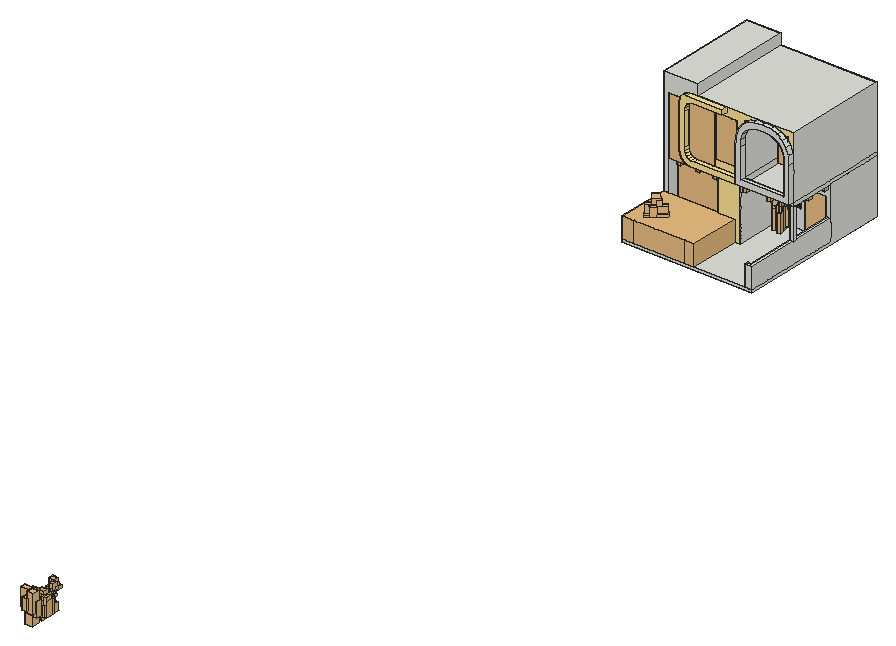
# SketchUp Ruby script. Lengths in inches.
U = 1.inch
M = Sketchup.active_model
def pt(a) = Geom::Point3d.new(a.map { |v| v * U })
def face(e, loops, mat)
  f = e.add_face(loops[0].map { |a| pt(a) })
  loops[1..].each { |l| e.add_face(l.map { |a| pt(a) }).erase! }
  f.material = f.back_material = mat if mat
  f
end
# faces: each face lists its corners as indices into pts; further lists are holes
def faces(e, pts, list, mat = nil) = list.each { |f| face(e, (f[0].is_a?(Array) ? f : [f]).map { |l| l.map { |i| pts[i] } }, mat) }
# xy, xz, yz: faces in a plane at the given z, y or x. An outline is a flat list of corners, or four numbers for a rectangle; further outlines are holes
def ring(l) = l.size == 4 ? [[l[0], l[1]], [l[2], l[1]], [l[2], l[3]], [l[0], l[3]]] : l.each_slice(2).to_a
def flat(e, list, mat, &to3) = list.each { |f| face(e, (f[0].is_a?(Array) ? f : [f]).map { |l| ring(l).map { |u, v| to3.(u, v) } }, mat) }
def xy(e, z, list, mat = nil) = flat(e, list, mat) { |x, y| [x, y, z] }
def xz(e, y, list, mat = nil) = flat(e, list, mat) { |x, z| [x, y, z] }
def yz(e, x, list, mat = nil) = flat(e, list, mat) { |y, z| [x, y, z] }
def lines(e, pts, list) = list.each { |a, b| e.add_line(pt(pts[a]), pt(pts[b])) }
# prism: a flat outline (further loops are holes) pulled along v
def prism(e, loops, v, mat = nil)
  f = face(e, loops, mat); d = Geom::Vector3d.new(v.map { |x| x * U })
  f.pushpull(f.normal.samedirection?(d) ? d.length : -d.length)
end
def box(e, o, s, mat = nil) = prism(e, [[o, [o[0] + s[0], o[1], o[2]], [o[0] + s[0], o[1] + s[1], o[2]], [o[0], o[1] + s[1], o[2]]]], [0, 0, s[2]], mat)
def at(x, y, z, deg = 0) = Geom::Transformation.translation(pt([x, y, z])) * Geom::Transformation.rotation(ORIGIN, Z_AXIS, deg.degrees)
def axes(o, x, y, z) = Geom::Transformation.new([*x, 0, *y, 0, *z, 0, *pt(o).to_a, 1])
def part(name) = M.definitions.add(name)
# library, detail: a bought-in or finely detailed component or shape, given as its bounding box
def library(name, o, s) = part(name).tap { |d| box(d.entities, o, s) }
def detail(e, o, s) = box(e.add_group.entities, o, s)
def put(e, d, t, mat = nil) = e.add_instance(d, t).tap { |i| i.material = mat if mat }
def group(e, t, mat = nil) = e.add_group.tap { |g| g.transformation = t; g.material = mat if mat }.entities
root = M.entities
M.materials.add("BANANA_BIG_STVOL_1").color = [93, 83, 53]
M.materials.add("Glass_Tinted_Gray").color = [0, 0, 0]
M.materials["Glass_Tinted_Gray"].alpha = 0.125
M.materials.add("POT_TEXTURE_1").color = [172, 172, 172]
M.materials.add("POT_TEXTURE_2").color = [160, 154, 144]
M.materials.add("[0135_DarkGray]").color = [81, 81, 81]
M.materials.add("[Color D02]").color = [255, 229, 153]
M.materials.add("[Mirror 02]").color = [229, 229, 229]
M.materials.add("[Terrazzo Light Blue]").color = [196, 214, 227]
M.materials.add("[Wood Veneer 02]").color = [190, 128, 91]
M.materials.add("soil1").color = [68, 55, 47]
M.materials.add("white_concrete_pot1").color = [212, 211, 204]
M.materials.add("wood_1").color = [140, 119, 94]
c1 = part("PENTEK_RP Fineline 50S_Sliding_DoorCase_E1")
box(c1.entities,[0,0,0],[1.51,3.66,99.27],"[0135_DarkGray]")
c2 = part("PENTEK_RP Fineline 50S_SlidingDooe_Case_E2")
box(c2.entities,[0,0,0],[96.25,3.66,1.51],"[0135_DarkGray]")
c3 = part("pentek_RP Fineline 50S_SlidingDoor_Case")
put(c3.entities,c1,at(97.76,0,0))
put(c3.entities,c2,at(1.51,0,0))
put(c3.entities,c1,at(0,0,0))
put(c3.entities,c2,at(1.51,0,97.76))
c4 = part("PENTEK_RP Fineline 50S_SlidingDoor_GlazingBead_2")
box(c4.entities,[0,0,0],[0.56,0.59,94.39],"[0135_DarkGray]")
c5 = part("PENTEK_RP Fineline 50S_SlidingDoor_Glass")
box(c5.entities,[0,0,0],[46.58,0.16,94.39],"Glass_Tinted_Gray")
c6 = part("PENTEK_RP Fineline 50S_SlidingDoor_GlazingBead")
box(c6.entities,[0,0,0],[45.47,0.59,0.56],"[0135_DarkGray]")
c7 = part("PENTEK_RP Fineline 50S_SlidingDoor_Leaf_E1")
xy(c7.entities,0,[[0,0,0.93,1.97],[0.93,1.57,1.49,1.97]],"[0135_DarkGray]")
xy(c7.entities,96.25,[[0,0,0.93,0,0.93,1.57,1.49,1.57,1.49,1.97,0,1.97]],"[0135_DarkGray]")
xz(c7.entities,0,[[0,0,0.93,96.25]],"[0135_DarkGray]")
xz(c7.entities,1.57,[[0.93,0,1.49,95.32],[0.93,95.32,1.49,96.25]],"[0135_DarkGray]")
xz(c7.entities,1.97,[[0,0,1.49,96.25]],"[0135_DarkGray]")
yz(c7.entities,0,[[0,0,1.97,96.25]],"[0135_DarkGray]")
yz(c7.entities,0.93,[[0,0,1.57,0.93],[0,0.93,1.57,95.32],[0,95.32,1.57,96.25]],"[0135_DarkGray]")
yz(c7.entities,1.49,[[1.57,0,1.97,95.32],[1.57,95.32,1.97,96.25]],"[0135_DarkGray]")
c8 = part("PENTEK_RP Fineline 50S_SlidingDoor_Leaf_E2")
xy(c8.entities,0,[[0,0,0,1.57,0.56,1.57,0.56,1.97,46.02,1.97,46.02,1.57,46.58,1.57,46.58,0]],"[0135_DarkGray]")
xy(c8.entities,0.93,[[0,0,46.58,1.57]],"[0135_DarkGray]")
xy(c8.entities,1.49,[[0.56,1.57,46.02,1.97]],"[0135_DarkGray]")
xz(c8.entities,0,[[0,0,46.58,0.93]],"[0135_DarkGray]")
xz(c8.entities,1.57,[[0,0,0.56,0.93],[46.02,0,46.58,0.93],[0.56,0.93,46.02,1.49]],"[0135_DarkGray]")
xz(c8.entities,1.97,[[0.56,0,46.02,1.49]],"[0135_DarkGray]")
yz(c8.entities,0,[[0,0,1.57,0.93]],"[0135_DarkGray]")
yz(c8.entities,0.56,[[1.57,0,1.97,0.93],[1.57,0.93,1.97,1.49]],"[0135_DarkGray]")
yz(c8.entities,46.02,[[1.57,0,1.97,0.93],[1.57,0.93,1.97,1.49]],"[0135_DarkGray]")
yz(c8.entities,46.58,[[0,0,1.57,0.93]],"[0135_DarkGray]")
c9 = part("PENTEK_RP Fineline S_SlidingDoor_Leaf1")
put(c9.entities,c4,at(0.93,0,0.93))
put(c9.entities,c4,at(46.96,0,0.93))
put(c9.entities,c5,at(1.49,1.42,0.93))
put(c9.entities,c6,at(1.49,0,0.93))
put(c9.entities,c5,at(1.49,0.59,0.93),"[Terrazzo Light Blue]")
put(c9.entities,c7,at(0,0,0))
put(c9.entities,c7,axes([48.44,0,0],[-1,0,0],[0,1,0],[0,0,1]))
put(c9.entities,c8,axes([0.93,0,96.25],[1,0,0],[0,1,0],[0,0,-1]))
put(c9.entities,c8,at(0.93,0,0))
put(c9.entities,c6,at(1.49,0,94.77))
c10 = part("PENTEK_RP Fineline 50S_SlidingDoor_Leaf2")
put(c10.entities,c5,at(1.49,1.42,0.93))
put(c10.entities,c6,at(1.49,0,94.77))
put(c10.entities,c4,at(46.96,0,0.93))
put(c10.entities,c5,at(1.49,0.59,0.93),"[Mirror 02]")
put(c10.entities,c4,at(0.93,0,0.93))
put(c10.entities,c7,at(0,0,0))
put(c10.entities,c7,axes([48.44,0,0],[-1,0,0],[0,1,0],[0,0,1]))
put(c10.entities,c6,at(1.49,0,0.93))
put(c10.entities,c8,axes([0.93,0,96.25],[1,0,0],[0,1,0],[0,0,-1]))
put(c10.entities,c8,at(0.93,0,0))
c11 = part("PENTEK - Slimmest Steel Sliding Door / Window\#1")
put(c11.entities,c3,at(0,-1.88,-0.09))
put(c11.entities,c9,at(1.51,-2.27,1.42))
put(c11.entities,c10,at(49.32,-0.3,1.42))
c12 = library("door by lz",[5.91,-4.92,0],[35.43,6.61,78.74])
c13 = library("Group14",[-64.97,9.24,0.31],[138.52,9.93,292.57])
c14 = library("Group16",[86.37,-10.76,76.46],[21.79,14.87,35.97])
c15 = library("Group22",[48.82,-10.91,0.23],[97.72,18.57,293.12])
c16 = library("Group24",[44.03,2.01,0.26],[103.73,11,292.35])
c17 = library("Group27",[-106.21,-10.76,76.46],[21.8,14.87,35.97])
c18 = library("Group35",[-145.81,2.01,0.26],[103.73,11,292.35])
c19 = library("Group33",[-144.59,-10.91,0.23],[97.72,18.57,293.12])
c20 = part("rem")
g1 = group(c20.entities,at(-145.81,-10.91,0.23))
put(g1,c13,at(145.81,10.91,-0.23))
put(g1,c14,at(145.81,10.91,-0.23))
put(g1,c15,at(145.81,10.91,-0.23))
put(g1,c16,at(145.81,10.91,-0.23))
put(g1,c17,at(145.81,10.91,-0.23))
put(g1,c18,at(145.81,10.91,-0.23))
put(g1,c19,at(145.81,10.91,-0.23))
c21 = library("Group\#9",[-312.76,2118.02,370.79],[80.37,61.43,57.53])
c22 = library("Group\#32",[-146.29,2044.53,349.125],[81,53.32,37.9])
c23 = library("Group\#76",[-236.03,2064.57,238.29],[378.97,266.89,1422.96])
c24 = library("Group\#19",[-392.38,2142.99,345.23],[79.77,60.6,39.05])
c25 = library("Group\#47",[-390.04,2074.71,363.78],[77.3,84.83,61.55])
c26 = library("Group\#23",[-389.63,2051.04,359.41],[56.81,81.38,37.86])
c27 = library("Group\#27",[-362.86,1963.26,351.01],[55.56,80.44,37.9])
c28 = library("Group\#31",[-200.52,1998.86,370.22],[77.15,68.38,35.39])
c29 = library("Group\#43",[-480.58,1843.32,11.96],[467.85,466.24,378.92])
c30 = library("Group\#20",[-433.57,2042.61,369.7],[71.79,72.8,37.85])
c31 = library("Group\#17",[-148.5,2084.1,354.63],[73.89,71.73,39.48])
c32 = library("Group\#57",[-372.4375,2154.5,374],[76.125,67.08,39.0625])
c33 = library("Group\#58",[-275.5,2156.34,352.11],[71.39,73.27,44.69])
c34 = library("Group\#37",[-143.56,2061.14,371.42],[79.79,63.19,51.3])
c35 = library("Group\#46",[-363.89,1895.22,354.63],[76.92,66.54,39.48])
c36 = library("Group\#39",[-145.08,2015.32,369.99],[82.29,54.05,37.9])
c37 = library("Group\#55",[-315.77,2202.04,371],[80.74,54.44,37.85])
c38 = library("Group\#48",[-419.21,1941.11,355.02],[73.1,71.21,39.06])
c39 = library("Group\#51",[-229.79,1894.04,351.01],[79.82,63.55,37.9])
c40 = library("Group\#63",[-234.26,2180.97,367.05],[50.63,74.65,43.95])
c41 = library("Group\#65",[-904.81,1865.01,156.3],[624.43,217.34,1227.7])
c42 = library("Group\#66",[-312.51,1611.52,263.78],[120.52,408.52,1275.1])
c43 = library("Group\#67",[-571.16,1736.08,232.33],[294.08,306.57,1438.75])
c44 = library("Group\#69",[-273.21,1593.22,47.51],[374.54,419.07,1416.6])
c45 = library("Group\#14",[-202.35,1900.5,372.29],[58.53,80.11,50.06])
c46 = library("Group\#22",[-432.01,1984.38,372.6875],[64.1,75.95,39.0625])
c47 = library("Group\#36",[-310.7,1952.62,354.63],[79.53,58.52,39.48])
c48 = library("Group\#21",[-374.28,1979.7,369.99],[51.81,82.66,37.9])
c49 = library("Group\#53",[-397.18,1916.74,372.44],[70.02,74.57,49.25])
c50 = library("Group\#60",[-236.3,2186.8,344.47],[79.26,62.91,39.06])
c51 = library("Group\#13",[-161.07,2117.49,373.61],[81.25,53.73,39.48])
c52 = library("Group\#64",[-431.9,1883.46,368.72],[373.65,376.39,18.61])
c53 = library("Group\#35",[-340.96,1970.4,361.28],[81.22,51.59,61.62])
c54 = library("Group\#41",[-272.7,1884.51,369.99],[80.39,55.87,37.9])
c55 = library("Group\#29",[-330.83,2117.69,370.2],[61.83,80.2,35.55])
c56 = library("Group\#62",[-366.3125,2177.8,359.41],[79.9,61.23,37.86])
c57 = library("Group\#26",[-435.875,2067.96,347.82],[58.32,80.53,38.29])
c58 = library("Group\#59",[-183.79,2161.45,371.25],[72.43,70.21,54.35])
c59 = library("Group\#68",[-208.23,2037.18,75.37],[621.09,225.61,1251.82])
c60 = library("Group\#71",[-675.58,1862.05,152.55],[378.81,196.01,1743.84])
c61 = library("Group\#72",[-257.06,2048.08,160.05],[394.6,177.93,1743.83])
c62 = library("Group\#73",[-344.84,1500.61,160.55],[176.35,551.19,1921.45])
c63 = library("Group\#74",[-231.77,1913.24,119.96],[448.93,143.84,1582.05])
c64 = library("Group\#75",[-616.67,2098.6,178.29],[331.19,111.16,1177.92])
c65 = library("Group\#70",[-527.15,2088.47,150.96],[267.01,328.12,1599.25])
c66 = library("Group\#77",[-792.12,2067.32,152.13],[549.56,259.52,1931.8])
c67 = library("Group\#78",[-281.17,2118.67,243.77],[133.23,408.71,1313.3])
c68 = part("Potted tropical plant")
g2 = group(c68.entities,at(904.81,-1500.61,-11.96),"white_concrete_pot1")
detail(g2,[-222.14,2117.95,372.07],[61.87,75.41,50.35])
put(c68.entities,c21,at(904.81,-1500.61,-11.96),"white_concrete_pot1")
g3 = group(c68.entities,at(904.81,-1500.61,-11.96),"white_concrete_pot1")
detail(g3,[-313.93,1881.02,351.21],[70.15,73.18,37.2])
g4 = group(c68.entities,at(904.81,-1500.61,-11.96),"white_concrete_pot1")
detail(g4,[-209.1,1970.26,378.89],[50.57,81.04,37.2])
put(c68.entities,c22,at(904.81,-1500.61,-11.96),"white_concrete_pot1")
put(c68.entities,c23,at(904.81,-1500.61,-11.96))
put(c68.entities,c24,at(904.81,-1500.61,-11.96),"white_concrete_pot1")
put(c68.entities,c25,at(904.81,-1500.61,-11.96),"white_concrete_pot1")
put(c68.entities,c26,at(904.81,-1500.61,-11.96),"white_concrete_pot1")
put(c68.entities,c27,at(904.81,-1500.61,-11.96),"white_concrete_pot1")
g5 = group(c68.entities,at(904.81,-1500.61,-11.96),"white_concrete_pot1")
detail(g5,[-129.49,1972.75,359.91],[55.59,80.76,37.2])
put(c68.entities,c28,at(904.81,-1500.61,-11.96),"white_concrete_pot1")
g6 = group(c68.entities,at(904.81,-1500.61,-11.96),"white_concrete_pot1")
detail(g6,[-333.13,1892.25,370.19],[61.39,79.4,37.2])
put(c68.entities,c29,at(904.81,-1500.61,-11.96),"POT_TEXTURE_1")
put(c68.entities,c30,at(904.81,-1500.61,-11.96),"white_concrete_pot1")
put(c68.entities,c31,at(904.81,-1500.61,-11.96),"white_concrete_pot1")
g7 = group(c68.entities,at(904.81,-1500.61,-11.96),"white_concrete_pot1")
detail(g7,[-270.91,2176.57,345.18],[52.11,82.01,38.29])
g8 = group(c68.entities,at(904.81,-1500.61,-11.96),"white_concrete_pot1")
detail(g8,[-195.71,2019.1875,371.11],[58.98,81.18,37.2])
g9 = group(c68.entities,at(904.81,-1500.61,-11.96),"white_concrete_pot1")
detail(g9,[-319.36,2078.81,339.18],[76.07,69.08,39.48])
put(c68.entities,c32,at(904.81,-1500.61,-11.96),"white_concrete_pot1")
put(c68.entities,c33,at(904.81,-1500.61,-11.96),"white_concrete_pot1")
g10 = group(c68.entities,at(904.81,-1500.61,-11.96),"white_concrete_pot1")
detail(g10,[-417.64,2112.53,369.82],[65.44,79.59,38.29])
put(c68.entities,c34,at(904.81,-1500.61,-11.96),"white_concrete_pot1")
put(c68.entities,c35,at(904.81,-1500.61,-11.96),"white_concrete_pot1")
put(c68.entities,c36,at(904.81,-1500.61,-11.96),"white_concrete_pot1")
g11 = group(c68.entities,at(904.81,-1500.61,-11.96),"white_concrete_pot1")
detail(g11,[-240.6,2054.85,378.89],[71.5,72.03,37.2])
put(c68.entities,c37,at(904.81,-1500.61,-11.96),"white_concrete_pot1")
put(c68.entities,c38,at(904.81,-1500.61,-11.96),"white_concrete_pot1")
put(c68.entities,c39,at(904.81,-1500.61,-11.96),"white_concrete_pot1")
g12 = group(c68.entities,at(904.81,-1500.61,-11.96),"white_concrete_pot1")
detail(g12,[-249.82,2117.53,359.91],[58.07,81.25,37.2])
put(c68.entities,c40,at(904.81,-1500.61,-11.96),"white_concrete_pot1")
put(c68.entities,c41,at(904.81,-1500.61,-11.96))
put(c68.entities,c42,at(904.81,-1500.61,-11.96))
put(c68.entities,c43,at(904.81,-1500.61,-11.96))
put(c68.entities,c44,at(904.81,-1500.61,-11.96))
g13 = group(c68.entities,at(904.81,-1500.61,-11.96),"white_concrete_pot1")
detail(g13,[-435.4375,2027.54,350.71],[78.74,62.6,37.86])
put(c68.entities,c45,at(904.81,-1500.61,-11.96),"white_concrete_pot1")
g14 = group(c68.entities,at(904.81,-1500.61,-11.96),"white_concrete_pot1")
detail(g14,[-173.8,2126.25,354.63],[80.17,60.53,39.48])
g15 = group(c68.entities,at(904.81,-1500.61,-11.96),"white_concrete_pot1")
detail(g15,[-222.96,2066.75,359.91],[63.77,78.21,37.2])
put(c68.entities,c46,at(904.81,-1500.61,-11.96),"white_concrete_pot1")
g16 = group(c68.entities,at(904.81,-1500.61,-11.96),"white_concrete_pot1")
detail(g16,[-183.125,1913.38,330.04],[66.78,77.69,39.48])
put(c68.entities,c47,at(904.81,-1500.61,-11.96),"white_concrete_pot1")
g17 = group(c68.entities,at(904.81,-1500.61,-11.96),"white_concrete_pot1")
detail(g17,[-152,1936.85,378.89],[64.46,79.76,37.2])
g18 = group(c68.entities,at(904.81,-1500.61,-11.96),"white_concrete_pot1")
detail(g18,[-284.65,1933.22,373.64],[80.83,55.23,37.2])
put(c68.entities,c48,at(904.81,-1500.61,-11.96),"white_concrete_pot1")
g19 = group(c68.entities,at(904.81,-1500.61,-11.96),"white_concrete_pot1")
detail(g19,[-263.49,1923.54,359.91],[75.98,66.75,37.2])
put(c68.entities,c49,at(904.81,-1500.61,-11.96),"white_concrete_pot1")
g20 = group(c68.entities,at(904.81,-1500.61,-11.96),"white_concrete_pot1")
detail(g20,[-167.97,1940.97,354.63],[66.78,77.7,39.48])
put(c68.entities,c50,at(904.81,-1500.61,-11.96),"white_concrete_pot1")
g21 = group(c68.entities,at(904.81,-1500.61,-11.96),"white_concrete_pot1")
detail(g21,[-214.75,1956.59,330.04],[66.78,77.69,39.48])
put(c68.entities,c51,at(904.81,-1500.61,-11.96),"white_concrete_pot1")
put(c68.entities,c52,at(904.81,-1500.61,-11.96),"white_concrete_pot1")
put(c68.entities,c53,at(904.81,-1500.61,-11.96),"white_concrete_pot1")
g22 = group(c68.entities,at(904.81,-1500.61,-11.96),"white_concrete_pot1")
detail(g22,[-282.5625,1934.21,389.56],[81.1,59.19,35.03])
put(c68.entities,c54,at(904.81,-1500.61,-11.96),"white_concrete_pot1")
g23 = group(c68.entities,at(904.81,-1500.61,-11.96),"white_concrete_pot1")
detail(g23,[-394.5,2036.48,359.91],[79.58,64.84,37.2])
put(c68.entities,c55,at(904.81,-1500.61,-11.96),"white_concrete_pot1")
put(c68.entities,c56,at(904.81,-1500.61,-11.96),"white_concrete_pot1")
put(c68.entities,c57,at(904.81,-1500.61,-11.96),"white_concrete_pot1")
put(c68.entities,c58,at(904.81,-1500.61,-11.96),"white_concrete_pot1")
put(c68.entities,c59,at(904.81,-1500.61,-11.96))
put(c68.entities,c60,at(904.81,-1500.61,-11.96))
put(c68.entities,c61,at(904.81,-1500.61,-11.96))
put(c68.entities,c62,at(904.81,-1500.61,-11.96))
put(c68.entities,c63,at(904.81,-1500.61,-11.96))
put(c68.entities,c64,at(904.81,-1500.61,-11.96))
put(c68.entities,c65,at(904.81,-1500.61,-11.96))
put(c68.entities,c66,at(904.81,-1500.61,-11.96))
put(c68.entities,c67,at(904.81,-1500.61,-11.96))
c69 = library("Group\#86",[-662.41,217.3,320.04],[397.32,658.3,1732.06])
c70 = library("Group\#88",[-299.2,181.55,262.58],[360.65,735.71,1258.34])
c71 = library("Group\#83",[-1038.76,656.55,345.34],[733.18,460.51,2065.7])
c72 = library("Group\#81",[-445.29,890.31,329.28],[284.3,304.08,2023.29])
c73 = library("Group\#84",[-733.48,439.625,202.64],[456.28,533.12,1536.78])
c74 = library("Group\#87",[-455.56,899.32,410.78],[341.21,610.33,1581.5])
c75 = library("Group\#80",[-516.34,626.77,-4.5625],[517.73,515.95,418.98])
c76 = library("Group\#85",[-249.24,914.85,310.18],[345.55,647.95,1307.93])
c77 = library("Group\#82",[-277.97,488.68,287.26],[362.84,405.94,1768.54])
c78 = library("Group\#79",[-468.76,669.89,380.1875],[424.36,427.47,41.99])
c79 = part("Potted broadleaf plant")
put(c79.entities,c69,at(1038.76,-181.55,4.5625))
put(c79.entities,c70,at(1038.76,-181.55,4.5625))
put(c79.entities,c71,at(1038.76,-181.55,4.5625))
put(c79.entities,c72,at(1038.76,-181.55,4.5625))
put(c79.entities,c73,at(1038.76,-181.55,4.5625))
put(c79.entities,c74,at(1038.76,-181.55,4.5625))
put(c79.entities,c75,at(1038.76,-181.55,4.5625),"POT_TEXTURE_1")
put(c79.entities,c76,at(1038.76,-181.55,4.5625))
put(c79.entities,c77,at(1038.76,-181.55,4.5625))
put(c79.entities,c78,at(1038.76,-181.55,4.5625),"soil1")
c80 = library("Group\#92",[-246.45,-349.05,558.47],[136.91,100.49,66.1])
c81 = library("Group\#95",[-264.68,-415.73,1484.11],[304.64,209.69,227.41])
c82 = library("Group\#102",[-357.04,-394.18,1447.05],[213.62,306.36,356.95])
c83 = library("Group\#90",[-447.02,-464.95,536.35],[343.73,346.24,39.39])
c84 = library("Group\#91",[-394.9,-448.99,911.74],[90.19,96.88,85.93])
c85 = library("Group\#101",[-424,-312.27,817.53],[158.81,108.06,136.45])
c86 = library("Group\#105",[-409.02,-515.05,915.53],[69.62,77.27,65.47])
c87 = library("Group\#109",[-548.25,-262.82,1459.54],[373.26,352.35,568])
c88 = library("Group\#116",[-492.14,-508.4,-4.15],[433.72,431.71,567.03])
c89 = library("Group\#112",[-293.78,-482.77,597.9],[158.75,112.78,159.87])
c90 = library("Group\#96",[-545.09,-386.51,922.3125],[300.25,219.65,227.33])
c91 = library("Group\#114",[-292.81,-667.38,1418.14],[215.17,356.07,188.87])
c92 = library("Group\#98",[-292.14,-288.9,1281.79],[169.55,204.34,203.36])
c93 = library("Group\#103",[-568.91,-444.37,1285.4],[307.6,179.39,277.93])
c94 = library("Group\#100",[-341.93,-403.49,744.8125],[64.83,96.32,132.15])
c95 = library("Group\#89",[-258.04,-282.68,604.05],[115.53,137.01,52.63])
c96 = library("Group\#97",[-304.79,-269.16,622.65],[82.06,111.89,102.57])
c97 = library("Group\#104",[-388.93,-514.39,838.93],[89.79,77.73,82.08])
c98 = library("Group\#106",[-295.03,-516.52,742.34],[68.71,141.75,78.67])
c99 = library("Group\#113",[-422.77,-235.4,843.61],[178.54,197.77,233.54])
c100 = library("Group\#107",[-498.98,-524.4,908.45],[120.83,107.95,112.98])
c101 = library("Group\#110",[-321.08,-139.66,1308.49],[285.55,393.29,221.53])
c102 = library("Group\#108",[-278.4,-571.99,1530.91],[311.57,345.77,423.62])
c103 = library("Group\#111",[-387.74,-136.11,1470.07],[230,321.58,230.27])
c104 = library("Group\#99",[-244.55,-305.59,1009.46],[103.13,76.81,77.34])
c105 = library("Group\#115",[-385.21,-446.52,494.02],[160.93,321.12,1142.36])
c106 = library("Group\#93",[-249.18,-250.59,980.93],[152.21,116.16,134.05])
c107 = library("Group\#94",[-438.92,-265.61,702.3],[171.52,146.16,133.5])
c108 = part("Potted broadleaf tree")
p = [[568.91,667.38,4.15],[569.91,667.38,4.15],[569.91,668.38,4.15]]
lines(c108.entities,p,[[0,1],[1,2],[2,0]])
put(c108.entities,c80,at(568.91,667.38,4.15))
put(c108.entities,c81,at(568.91,667.38,4.15))
put(c108.entities,c82,at(568.91,667.38,4.15))
put(c108.entities,c83,at(568.91,667.38,4.15),"soil1")
put(c108.entities,c84,at(568.91,667.38,4.15))
put(c108.entities,c85,at(568.91,667.38,4.15))
put(c108.entities,c86,at(568.91,667.38,4.15))
put(c108.entities,c87,at(568.91,667.38,4.15))
put(c108.entities,c88,at(568.91,667.38,4.15),"POT_TEXTURE_2")
put(c108.entities,c89,at(568.91,667.38,4.15))
put(c108.entities,c90,at(568.91,667.38,4.15))
put(c108.entities,c91,at(568.91,667.38,4.15))
put(c108.entities,c92,at(568.91,667.38,4.15))
put(c108.entities,c93,at(568.91,667.38,4.15))
put(c108.entities,c94,at(568.91,667.38,4.15))
put(c108.entities,c95,at(568.91,667.38,4.15))
put(c108.entities,c96,at(568.91,667.38,4.15))
put(c108.entities,c97,at(568.91,667.38,4.15))
put(c108.entities,c98,at(568.91,667.38,4.15))
put(c108.entities,c99,at(568.91,667.38,4.15))
put(c108.entities,c100,at(568.91,667.38,4.15))
put(c108.entities,c101,at(568.91,667.38,4.15))
put(c108.entities,c102,at(568.91,667.38,4.15))
put(c108.entities,c103,at(568.91,667.38,4.15))
put(c108.entities,c104,at(568.91,667.38,4.15))
put(c108.entities,c105,at(568.91,667.38,4.15),"wood_1")
put(c108.entities,c106,at(568.91,667.38,4.15))
put(c108.entities,c107,at(568.91,667.38,4.15))
c109 = library("Group\#127",[-640.625,-1318.37,287.11],[396.64,314.81,689.96])
c110 = library("Group\#119",[-513.94,-1201.2,195.17],[480.66,557.42,1160.08])
c111 = library("Group\#121",[-208.03,-1336.63,286.21],[381.72,484.79,1145.39])
c112 = library("Group\#130",[-619.83,-1636.3,288.9],[316.15,456.61,1171.28])
c113 = library("Group\#131",[-738.91,-1210.08,301],[426.4,388.88,1000.79])
c114 = library("Group\#133",[-208.33,-1511.76,297.04],[508.2,421.96,1258.76])
c115 = library("Group\#120",[-545.36,-1775.03,287.125],[412.21,432,920.68])
c116 = library("Group\#128",[-750.24,-1478.51,301.56],[423.84,451.05,998.69])
c117 = library("Group\#123",[-245.33,-1174.2,301.22],[356.02,306.31,608.34])
c118 = library("Group\#118",[-487.23,-1483.58,-4.71],[450.86,446.99,418.38])
c119 = library("Group\#135",[-445.7,-1606.55,154.18],[255.44,283.57,849.28])
c120 = library("Group\#136",[-390.1,-1177.12,195.59],[220.93,265.44,790.12])
c121 = library("Group\#138",[-480.32,-1333.42,295.8],[424.49,356.06,1482.77])
c122 = library("Group\#139",[-378.01,-1245.98,305.66],[422.15,474.55,1267.42])
c123 = library("Group\#122",[-163.65,-1622.09,292.29],[406.18,374.8,780.12])
c124 = library("Group\#134",[-384.8,-1640.99,300.61],[422.68,348.03,1297.96])
c125 = library("Group\#117",[-429.18,-1441.17,362.05],[345.84,348.28,45.35])
c126 = library("Group\#137",[-208.0625,-1498.77,286.27],[547.26,435.76,1075.6])
c127 = library("Group\#132",[-172.82,-1329.68,294.68],[502.85,397.72,955.79])
c128 = library("Group\#129",[-426.76,-1753.59,287.48],[479.67,412.35,1049.19])
c129 = part("Potted palm")
put(c129.entities,c109,at(750.24,1775.03,4.71))
put(c129.entities,c110,at(750.24,1775.03,4.71))
put(c129.entities,c111,at(750.24,1775.03,4.71))
put(c129.entities,c112,at(750.24,1775.03,4.71))
put(c129.entities,c113,at(750.24,1775.03,4.71))
put(c129.entities,c114,at(750.24,1775.03,4.71))
put(c129.entities,c115,at(750.24,1775.03,4.71))
put(c129.entities,c116,at(750.24,1775.03,4.71))
put(c129.entities,c117,at(750.24,1775.03,4.71))
put(c129.entities,c118,at(750.24,1775.03,4.71),"POT_TEXTURE_1")
put(c129.entities,c119,at(750.24,1775.03,4.71))
put(c129.entities,c120,at(750.24,1775.03,4.71))
put(c129.entities,c121,at(750.24,1775.03,4.71))
put(c129.entities,c122,at(750.24,1775.03,4.71))
put(c129.entities,c123,at(750.24,1775.03,4.71))
put(c129.entities,c124,at(750.24,1775.03,4.71))
put(c129.entities,c125,at(750.24,1775.03,4.71),"soil1")
put(c129.entities,c126,at(750.24,1775.03,4.71))
put(c129.entities,c127,at(750.24,1775.03,4.71))
put(c129.entities,c128,at(750.24,1775.03,4.71))
c130 = library("Group\#140",[-480.3,-2300.47,677.45],[398.14,398.43,28.25])
c131 = library("Group\#141",[-336.38,-2175.79,614.41],[133.99,147.1,560.64])
c132 = library("Group\#142",[-311.45,-2362.85,663.67],[597.01,322.07,1007.38])
c133 = library("Group\#143",[-330.26,-2159.14,612.04],[116.66,119.22,673.97])
c134 = library("Group\#144",[-667.53,-2111.4375,1071.74],[420.02,555.28,968.03])
c135 = library("Group\#145",[-328.97,-2115.58,1156.29],[117.86,119.42,695.38])
c136 = library("Group\#146",[-943.22,-2312.1875,967.59],[670.63,402.45,1245.73])
c137 = library("Group\#148",[-343.93,-2076.42,1024.91],[285.05,475.82,708.21])
c138 = library("Group\#147",[-568.09,-2386.9,-3.76],[573.62,569.18,700.28])
c139 = library("Group\#149",[-550.09,-2664.39,1031.96],[371.42,533.86,798])
c140 = library("Group\#150",[-308.37,-2556.11,869.35],[483.58,483.6,1385.8])
c141 = part("Potted broadleaf plant \#1")
put(c141.entities,c130,at(943.22,2664.39,3.76),"soil1")
put(c141.entities,c131,at(943.22,2664.39,3.76),"BANANA_BIG_STVOL_1")
put(c141.entities,c132,at(943.22,2664.39,3.76))
put(c141.entities,c133,at(943.22,2664.39,3.76),"BANANA_BIG_STVOL_1")
put(c141.entities,c134,at(943.22,2664.39,3.76))
put(c141.entities,c135,at(943.22,2664.39,3.76))
put(c141.entities,c136,at(943.22,2664.39,3.76))
put(c141.entities,c137,at(943.22,2664.39,3.76))
put(c141.entities,c138,at(943.22,2664.39,3.76),"POT_TEXTURE_2")
put(c141.entities,c139,at(943.22,2664.39,3.76))
put(c141.entities,c140,at(943.22,2664.39,3.76))
c142 = part("plants(2)")
put(c142.entities,c68,at(3946.86,59449.77,327.96,-71))
put(c142.entities,c79,at(-1226.73,54039.72,327.96,-50.633))
put(c142.entities,c108,at(-568.91,-667.38,-4.15))
put(c142.entities,c129,at(-750.24,-1775.03,-4.71))
put(c142.entities,c141,at(-943.22,-2664.39,-3.76))
put(c142.entities,c79,at(5933.24,59573.55,4303.12,-87.233))
c143 = part("Group374\#1")
p = [[0,0,0],[0,0,-7.72],[-0.15,0,-7.72],[1,-24,0],[-1,-24,0],[1,24,0],
  [1,0,0],[-1,24,0],[0.15,0,-7.72],[-1,0,0],[0,0,-12.5]]
lines(c143.entities,p,[[0,1],[1,2],[3,4],[5,6],[7,5],[1,8],[9,0],[0,6],[8,10],[4,9],[6,3],[2,10],
  [9,7]])
c144 = part("Rectangle Light\#3")
put(c144.entities,c143,at(0,0,0))
c145 = part("Group376\#1")
p = [[0,0,0],[0,0,-7.72],[-0.15,0,-7.72],[1,-24,0],[-1,-24,0],[1,24,0],
  [1,0,0],[-1,24,0],[0.15,0,-7.72],[-1,0,0],[0,0,-12.5]]
lines(c145.entities,p,[[0,1],[1,2],[3,4],[5,6],[7,5],[1,8],[9,0],[0,6],[8,10],[4,9],[6,3],[2,10],
  [9,7]])
c146 = part("Rectangle Light\#4")
put(c146.entities,c145,at(0,0,0))
c147 = library("IES Light",[-4.45,-4.45,-12],[8.9,8.9,12])
c148 = library("Sliding windows",[297.42,-0.89,0.35],[194.88,8.85,122.84])
c149 = library("шторы раздвинутые\#1",[23.6875,-79.37,-3.6],[68.3125,79.85,10.87])
c150 = part("Group383\#1")
p = [[0,0,0],[0,0,-17.77],[-8.76,0,-17.77],[57.04,-0.5,0],[-57.04,-0.5,0],[57.04,0.5,0],
  [57.04,0,0],[-57.04,0.5,0],[8.76,0,-17.77],[-57.04,0,0],[0,0,-28.77]]
lines(c150.entities,p,[[0,1],[1,2],[3,4],[5,6],[7,5],[1,8],[9,0],[0,6],[8,10],[4,9],[6,3],[2,10],
  [9,7]])
c151 = part("Rectangle Light\#5")
put(c151.entities,c150,at(0,0,0))
c152 = part("Group385\#1")
p = [[0,0,0],[0,0,-15.78],[-7.77,0,-15.78],[50.6,-0.5,0],[-50.6,-0.5,0],[50.6,0.5,0],
  [50.6,0,0],[-50.6,0.5,0],[7.77,0,-15.78],[-50.6,0,0],[0,0,-25.55]]
lines(c152.entities,p,[[0,1],[1,2],[3,4],[5,6],[7,5],[1,8],[9,0],[0,6],[8,10],[4,9],[6,3],[2,10],
  [9,7]])
c153 = part("Rectangle Light\#6")
put(c153.entities,c152,at(0,0,0))
c154 = library("Group2\#1",[-50.56,-64.53,0],[101.12,129.06,0.24])
c155 = library("Group106\#2",[-30.52,-60,0],[61,120,0.25])
c156 = library("Group128\#2",[-17.41,-67.375,0],[34.82,134.75,0.25])
c157 = library("Group\#4",[-0.5,-0.5,-0.1],[49,97,0.2])
c158 = library("Group\#152",[-0.5,-0.5,-0.1],[94.22,80.42,0.2])
c159 = library("Group\#6",[0,0,0],[166.2,120,48])
put(root,c11,axes([183.2,231.61,48.39],[0.48352,0,0],[0,0.3,0],[0,0,0.48444]))
put(root,c12,axes([231.99,233.42,6],[1.35467,0,0],[0,1,0],[0,0,1.14856]))
put(root,c20,axes([68.66,160.48,5.91],[0.38859,0,0],[0,0.26,0],[0,0,0.40939]))
put(root,c142,axes([49.51,-1690.71,-4.56],[0.0322,0,0],[0,0.0322,0],[0,0,0.0322]))
put(root,c144,axes([144.1875,1,30],[0,-1,0],[0,0,1],[1,0,0]))
put(root,c146,axes([26.45,1,30],[0,-1,0],[0,0,-1],[-1,0,0]))
put(root,c147,at(185.8,127.6,125.99))
put(root,c147,at(185.8,220.23,125.99))
put(root,c147,at(185.8,173.8,125.99))
put(root,c147,at(292.23,220.23,125.99))
put(root,c147,at(292.23,173.8,125.99))
put(root,c147,at(288.98,127.6,125.99))
put(root,c147,at(239.73,220.23,125.99))
put(root,c147,at(239.73,127.6,125.99))
put(root,c147,at(194.24,211.14,265.79))
put(root,c147,at(278.06,211.14,265.79))
put(root,c147,at(233.81,211.14,265.79))
put(root,c147,at(278.06,136.96,265.79))
put(root,c147,at(194.24,136.96,265.79))
put(root,c147,at(233.81,135.11,265.79))
put(root,c147,at(194.24,174.33,265.79))
put(root,c147,at(278.06,175.33,265.79))
put(root,c147,at(112.25,131.76,126))
put(root,c147,at(72.13,131.76,126))
put(root,c147,at(29.27,131.76,126))
g24 = group(root,at(0,0,0))
xy(g24,0,[[0,0,300,360]])
xy(g24,6,[[0,0,300,0,300,228,288,228,288,239.8125,240,239.8125,240,228,178.2,228,178.2,117.625,126.08,117.625,126.08,228,12,228,12,120,0,120],[126.08,117.625,178.2,120]])
xy(g24,48.4375,[[183.2,228,231.2,239.8125]])
xy(g24,96.4375,[[183.2,228,231.2,239.8125],[240,228,288,239.8125]])
xy(g24,126,[[12,120,126.08,142.89],[[178.2,120,300,228],[192.49,134.29,285.71,213.71]],[193.2,135,285,213],[12,142.89,126.08,228]])
xy(g24,134,[[174.88,108,174.88,117.625,178.2,117.625,178.2,120,300,120,300,108],[126.08,117.625,174.88,120],[174.88,117.625,178.2,120],[186.88,120,288,261.9375]])
xy(g24,134,[[71.23,108,71.64,120],[71.64,108,71.64,120,126.08,120,126.08,117.625,174.88,117.625,174.88,108]],"[Color D02]")
xy(g24,146,[[186.88,108,288,120]])
xy(g24,146,[[79.95,108,174.88,120]],"[Color D02]")
xy(g24,266,[[79.95,108,144.93,120]],"[Color D02]")
xy(g24,278,[[237.29,108,237.59,120],[78.34,120,300,360]])
xy(g24,278,[[63.89,108,144.93,120]],"[Color D02]")
xy(g24,302,[[0,120,78.34,360]])
xz(g24,0,[[0,0,300,6]])
xz(g24,108,[[[174.88,134,300,134,300,215.59,298.27,234.66,293.07,250.26,284.4,262.4,272.26,271.07,256.66,276.27,237.59,278,237.29,278,218.22,276.27,202.62,271.07,190.49,262.4,181.82,250.26,176.62,234.66,174.88,215.59],[186.88,146,186.88,215.24,188.29,230.68,192.5,243.32,199.52,253.15,209.35,260.18,221.99,264.39,237.44,265.79,252.89,264.39,265.53,260.18,275.36,253.15,282.38,243.32,286.6,230.68,288,215.24,288,146]]])
xz(g24,108,[[71.23,134,174.88,134,174.88,146,79.95,146,73.05,146.63,67.41,148.51,63.02,151.64,59.88,156.03,58,161.68,57.375,168.57,57.375,243.43,58,250.32,59.88,255.97,63.02,260.36,67.41,263.49,73.05,265.37,79.95,266,144.93,266,144.93,278,63.89,278,58.23,277.49,53.61,275.94,50,273.37,47.43,269.77,45.89,265.14,45.375,259.48,45.375,160.27,45.38,159.86,45.39,159.44,45.4,159.03,45.49,157.8,45.53,157.39,45.58,156.98,45.7,156.16,45.77,155.75,45.84,155.35,45.92,154.94,46.1,154.14,46.2,153.74,46.42,152.94,46.54,152.55,46.66,152.15,46.79,151.76,47.07,150.98,47.22,150.6,47.375,150.22,47.54,149.84,47.7,149.46,47.875,149.08,48.05,148.71,48.24,148.34,48.43,147.98,48.625,147.61,48.83,147.25,49.03,146.9,49.25,146.54,49.46,146.19,49.6875,145.85,49.92,145.5,50.15,145.16,50.39,144.83,51.14,143.84,51.4,143.52,51.67,143.21,51.9375,142.9,52.21,142.59,52.49,142.29,53.07,141.69,53.36,141.4,53.96,140.84,54.27,140.5625,54.58,140.29,55.54,139.51,55.87,139.26,56.2,139.02,56.88,138.54,57.22,138.3125,57.57,138.09,57.92,137.87,58.27,137.66,58.63,137.45,59.35,137.05,59.72,136.86,60.46,136.5,60.83,136.33,61.21,136.16,61.97,135.84,62.36,135.7,62.75,135.55,63.92,135.16,64.32,135.04,64.71,134.93,65.91,134.63,66.32,134.55,66.72,134.47,67.13,134.39,67.53,134.32,67.94,134.26,68.76,134.16,69.58,134.08,69.99,134.05,70.41,134.03,70.82,134.01]],"[Color D02]")
xz(g24,117.625,[[126.08,6,178.2,134]],"[Color D02]")
xz(g24,120,[[0,6,12,6,12,260.75,45.49,260.75,45.89,265.14,47.43,269.77,50,273.37,53.61,275.94,58.23,277.49,63.89,278,78.34,278,78.34,302,0,302],[126.08,6,178.2,134],[46.8125,126,126.08,126,126.08,134,71.23,134,70.82,134.01,70.41,134.03,69.99,134.05,69.58,134.08,68.76,134.16,67.94,134.26,67.53,134.32,67.13,134.39,66.72,134.47,66.32,134.55,65.91,134.63,64.71,134.93,64.32,135.04,63.92,135.16,62.75,135.55,62.36,135.7,61.97,135.84,61.21,136.16,60.83,136.33,60.46,136.5,59.72,136.86,59.35,137.05,58.63,137.45,58.27,137.66,57.92,137.87,57.57,138.09,57.22,138.3125,56.88,138.54,56.2,139.02,55.87,139.26,55.54,139.51,54.58,140.29,54.27,140.5625,53.96,140.84,53.36,141.4,53.07,141.69,52.49,142.29,52.21,142.59,51.9375,142.9,51.67,143.21,51.4,143.52,51.14,143.84,50.39,144.83,50.15,145.16,49.92,145.5,49.6875,145.85,49.46,146.19,49.25,146.54,49.03,146.9,48.83,147.25,48.625,147.61,48.43,147.98,48.24,148.34,48.05,148.71,47.875,149.08,47.7,149.46,47.54,149.84,47.375,150.22,47.22,150.6,47.07,150.98,46.93,151.37,46.8125,151.7],[178.2,126,300,134],[71.23,134,174.88,134,174.88,146,79.95,146,73.05,146.63,67.41,148.51,63.02,151.64,59.88,156.03,58,161.68,57.375,168.57,57.375,243.43,58,250.32,59.88,255.97,63.02,260.36,67.41,263.49,73.05,265.37,79.95,266,144.93,266,144.93,278,63.89,278,58.23,277.49,53.61,275.94,50,273.37,47.43,269.77,45.89,265.14,45.49,260.75,46.8125,260.75,46.8125,151.7,46.93,151.37,47.07,150.98,47.22,150.6,47.375,150.22,47.54,149.84,47.7,149.46,47.875,149.08,48.05,148.71,48.24,148.34,48.43,147.98,48.625,147.61,48.83,147.25,49.03,146.9,49.25,146.54,49.46,146.19,49.6875,145.85,49.92,145.5,50.15,145.16,50.39,144.83,51.14,143.84,51.4,143.52,51.67,143.21,51.9375,142.9,52.21,142.59,52.49,142.29,53.07,141.69,53.36,141.4,53.96,140.84,54.27,140.5625,54.58,140.29,55.54,139.51,55.87,139.26,56.2,139.02,56.88,138.54,57.22,138.3125,57.57,138.09,57.92,137.87,58.27,137.66,58.63,137.45,59.35,137.05,59.72,136.86,60.46,136.5,60.83,136.33,61.21,136.16,61.97,135.84,62.36,135.7,62.75,135.55,63.92,135.16,64.32,135.04,64.71,134.93,65.91,134.63,66.32,134.55,66.72,134.47,67.13,134.39,67.53,134.32,67.94,134.26,68.76,134.16,69.58,134.08,69.99,134.05,70.41,134.03,70.82,134.01],
  [186.88,134,288,146],[46.8125,151.7,46.8125,260.75,45.49,260.75,45.375,259.48,45.375,160.27,45.38,159.86,45.39,159.44,45.4,159.03,45.49,157.8,45.53,157.39,45.58,156.98,45.7,156.16,45.77,155.75,45.84,155.35,45.92,154.94,46.1,154.14,46.2,153.74,46.42,152.94,46.54,152.55,46.66,152.15,46.79,151.76],[186.88,215.24,186.88,257.36,190.49,262.4,195.24,265.79,237.44,265.79,221.99,264.39,209.35,260.18,199.52,253.15,192.5,243.32,188.29,230.68],[288,215.24,286.6,230.68,282.38,243.32,275.36,253.15,265.53,260.18,252.89,264.39,237.44,265.79,279.64,265.79,284.4,262.4,288,257.36]])
xz(g24,120,[[118.42,146,174.88,146,174.88,215.59,176.62,234.66,181.82,250.26,186.88,257.36,186.88,265.79,195.24,265.79,202.62,271.07,218.22,276.27,237.29,278,144.93,278,144.93,266,118.42,266],[300,215.59,300,278,237.59,278,256.66,276.27,272.26,271.07,279.64,265.79,288,265.79,288,257.36,293.07,250.26,298.27,234.66],[186.88,257.36,190.49,262.4,195.24,265.79,186.88,265.79],[288,257.36,288,265.79,279.64,265.79,284.4,262.4]],"[Color D02]")
xz(g24,228,[[12,6,126.08,126],[[178.2,6,240,6,240,96.4375,288,96.4375,288,6,300,6,300,126,178.2,126],[183.2,48.4375,231.2,96.4375]]])
xz(g24,239.8125,[[240,6,288,96.4375],[183.2,48.4375,231.2,96.4375]])
xz(g24,261.9375,[[186.88,134,288,265.79]])
xz(g24,360,[[0,0,300,126],[0,126,300,134],[0,134,0,302,78.34,302,78.34,278,300,278,300,134]])
yz(g24,0,[[0,0,0,6,120,6,120,126,360,126,360,0],[120,126,360,134],[120,134,360,302]])
yz(g24,12,[[120,6,146.27,126],[146.27,6,228,126]])
yz(g24,45.375,[[108,160.27,120,259.48]],"[Color D02]")
yz(g24,57.375,[[108,168.57,120,243.43]],"[Color D02]")
yz(g24,78.34,[[120,278,360,302]])
yz(g24,126.08,[[120,6,142.89,126],[142.89,6,228,126]])
yz(g24,126.08,[[117.625,6,120,134]],"[Color D02]")
yz(g24,144.93,[[108,266,120,278]],"[Color D02]")
yz(g24,174.88,[[108,134,120,146],[108,146,120,215.59]])
yz(g24,178.2,[[120,6,228,126]])
yz(g24,178.2,[[117.625,6,120,134]],"[Color D02]")
yz(g24,183.2,[[228,48.4375,239.8125,96.4375]])
yz(g24,186.88,[[120,134,261.9375,146],[108,146,120,215.24],[120,146,261.9375,265.79]])
yz(g24,231.2,[[228,48.4375,239.8125,96.4375]])
yz(g24,240,[[228,6,239.8125,96.4375]])
yz(g24,288,[[228,6,239.8125,96.4375],[120,134,261.9375,265.79],[108,146,120,215.24]])
yz(g24,300,[[0,0,360,0,360,126,228,126,228,6,0,6],[120,126,360,134],[108,134,120,215.59],[120,134,360,278]])
p = [[70.41,108,134.03],[69.99,108,134.05],[69.99,120,134.05],[70.41,120,134.03],[70.82,108,134.01],[70.82,120,134.01],
  [71.23,108,134],[71.23,120,134],[69.17,108,134.12],[68.76,108,134.16],[68.76,120,134.16],[69.17,120,134.12],
  [69.58,108,134.08],[69.58,120,134.08],[68.35,108,134.21],[67.94,108,134.26],[67.94,120,134.26],[68.35,120,134.21],
  [67.53,108,134.32],[67.13,108,134.39],[67.13,120,134.39],[67.53,120,134.32],[66.72,108,134.47],[66.72,120,134.47],
  [66.32,108,134.55],[65.91,108,134.63],[65.91,120,134.63],[66.32,120,134.55],[65.51,108,134.73],[65.51,120,134.73],
  [65.11,108,134.83],[65.11,120,134.83],[64.71,108,134.93],[64.71,120,134.93],[64.32,108,135.04],[64.32,120,135.04],
  [63.92,108,135.16],[63.92,120,135.16],[63.53,108,135.29],[63.53,120,135.29],[63.14,108,135.42],[63.14,120,135.42],
  [62.75,108,135.55],[62.75,120,135.55],[62.36,108,135.7],[62.36,120,135.7],[61.97,108,135.84],[61.97,120,135.84],
  [61.59,108,136],[61.59,120,136],[61.21,108,136.16],[61.21,120,136.16],[60.83,108,136.33],[60.83,120,136.33],
  [60.46,108,136.5],[60.46,120,136.5],[60.09,108,136.68],[60.09,120,136.68],[59.72,108,136.86],[59.72,120,136.86],
  [59.35,108,137.05],[59.35,120,137.05],[58.99,108,137.25],[58.99,120,137.25],[58.63,108,137.45],[58.63,120,137.45],
  [58.27,108,137.66],[58.27,120,137.66],[57.92,108,137.87],[57.92,120,137.87],[57.57,108,138.09],[57.57,120,138.09],
  [57.22,108,138.3125],[57.22,120,138.3125],[56.88,108,138.54],[56.88,120,138.54],[56.54,108,138.78],[56.54,120,138.78],
  [56.2,108,139.02],[56.2,120,139.02],[55.87,108,139.26],[55.87,120,139.26],[55.54,108,139.51],[55.54,120,139.51],
  [55.22,108,139.77],[55.22,120,139.77],[54.9,108,140.03],[54.9,120,140.03],[54.58,108,140.29],[54.58,120,140.29],
  [54.27,108,140.5625],[54.27,120,140.5625],[53.96,108,140.84],[53.96,120,140.84],[53.66,108,141.12],[53.66,120,141.12],
  [53.36,108,141.4],[53.36,120,141.4],[53.07,108,141.69],[53.07,120,141.69],[52.78,108,141.99],[52.78,120,141.99],
  [52.49,108,142.29],[52.49,120,142.29],[52.21,108,142.59],[52.21,120,142.59],[51.9375,108,142.9],[51.9375,120,142.9],
  [51.67,108,143.21],[51.67,120,143.21],[51.4,108,143.52],[51.4,120,143.52],[51.14,108,143.84],[51.14,120,143.84],
  [50.89,108,144.17],[50.89,120,144.17],[50.64,108,144.5],[50.64,120,144.5],[50.39,108,144.83],[50.39,120,144.83],
  [50.15,108,145.16],[50.15,120,145.16],[49.92,108,145.5],[49.92,120,145.5],[49.6875,108,145.85],[49.6875,120,145.85],
  [49.46,108,146.19],[49.46,120,146.19],[79.95,108,146],[79.95,120,146],[73.05,120,146.63],[73.05,108,146.63],
  [49.25,108,146.54],[49.25,120,146.54],[49.03,108,146.9],[49.03,120,146.9],[67.41,120,148.51],[67.41,108,148.51],
  [48.83,108,147.25],[48.83,120,147.25],[48.625,108,147.61],[48.625,120,147.61],[48.43,108,147.98],[48.43,120,147.98],
  [48.24,108,148.34],[48.24,120,148.34],[48.05,108,148.71],[48.05,120,148.71],[63.02,120,151.64],[63.02,108,151.64],
  [47.875,108,149.08],[47.875,120,149.08],[47.7,108,149.46],[47.7,120,149.46],[47.54,108,149.84],[47.54,120,149.84],
  [47.375,108,150.22],[47.375,120,150.22],[47.22,108,150.6],[47.22,120,150.6],[47.07,108,150.98],[47.07,120,150.98],
  [46.93,108,151.37],[46.93,120,151.37],[46.79,108,151.76],[46.79,120,151.76],[46.8125,120,151.7],[59.88,120,156.03],
  [59.88,108,156.03],[46.66,108,152.15],[46.66,120,152.15],[46.54,108,152.55],[46.54,120,152.55],[46.42,108,152.94],
  [46.42,120,152.94],[46.31,108,153.34],[46.31,120,153.34],[46.2,108,153.74],[46.2,120,153.74],[46.1,108,154.14],
  [46.1,120,154.14],[46.01,108,154.54],[46.01,120,154.54],[45.92,108,154.94],[45.92,120,154.94],[45.84,108,155.35],
  [45.84,120,155.35],[45.77,108,155.75],[45.77,120,155.75],[45.7,108,156.16],[45.7,120,156.16],[58,120,161.68],
  [58,108,161.68],[45.64,108,156.57],[45.64,120,156.57],[45.58,108,156.98],[45.58,120,156.98],[45.53,108,157.39],
  [45.53,120,157.39],[45.49,108,157.8],[45.49,120,157.8],[45.46,108,158.21],[45.46,120,158.21],[45.43,108,158.62],
  [45.43,120,158.62],[45.4,108,159.03],[45.4,120,159.03],[45.39,108,159.44],[45.39,120,159.44],[45.38,108,159.86],
  [45.38,120,159.86],[45.375,108,160.27],[45.375,120,160.27],[57.375,120,168.57],[57.375,108,168.57],[188.29,120,230.68],
  [188.29,108,230.68],[186.88,108,215.24],[186.88,120,215.24],[288,120,215.24],[288,108,215.24],[286.6,108,230.68],
  [286.6,120,230.68],[174.88,120,215.59],[174.88,108,215.59],[176.62,108,234.66],[176.62,120,234.66],[300,108,215.59],
  [300,120,215.59],[298.27,120,234.66],[298.27,108,234.66],[192.5,120,243.32],[192.5,108,243.32],[282.38,108,243.32],
  [282.38,120,243.32],[181.82,108,250.26],[181.82,120,250.26],[293.07,120,250.26],[293.07,108,250.26],[199.52,120,253.15],
  [199.52,108,253.15],[275.36,108,253.15],[275.36,120,253.15],[58,120,250.32],[58,108,250.32],[57.375,108,243.43],
  [57.375,120,243.43],[59.88,120,255.97],[59.88,108,255.97],[190.49,108,262.4],[190.49,120,262.4],[186.88,120,257.36],
  [288,120,257.36],[284.4,120,262.4],[284.4,108,262.4],[209.35,120,260.18],[209.35,108,260.18],[265.53,108,260.18],
  [265.53,120,260.18],[63.02,120,260.36],[63.02,108,260.36],[45.375,120,259.48],[45.375,108,259.48],[45.89,108,265.14],
  [45.89,120,265.14],[45.49,120,260.75],[221.99,120,264.39],[221.99,108,264.39],[252.89,108,264.39],[252.89,120,264.39],
  [67.41,120,263.49],[67.41,108,263.49],[202.62,108,271.07],[202.62,120,271.07],[195.24,120,265.79],[279.64,120,265.79],
  [272.26,120,271.07],[272.26,108,271.07],[73.05,120,265.37],[73.05,108,265.37],[237.44,120,265.79],[237.44,108,265.79],
  [47.43,108,269.77],[47.43,120,269.77],[79.95,120,266],[79.95,108,266],[50,108,273.37],[50,120,273.37],
  [218.22,108,276.27],[218.22,120,276.27],[256.66,120,276.27],[256.66,108,276.27],[53.61,108,275.94],[53.61,120,275.94],
  [58.23,108,277.49],[58.23,120,277.49],[237.29,108,278],[237.29,120,278],[237.59,120,278],[237.59,108,278],
  [63.89,108,278],[63.89,120,278]]
faces(g24,p,[[0,1,2,3],[4,0,3,5],[6,4,5,7],[8,9,10,11],[12,8,11,13],[1,12,13,2],[14,15,16,17],[9,14,17,10],
  [18,19,20,21],[15,18,21,16],[19,22,23,20],[24,25,26,27],[22,24,27,23],[25,28,29,26],[28,30,31,29],[30,32,33,31],
  [32,34,35,33],[34,36,37,35],[36,38,39,37],[38,40,41,39],[40,42,43,41],[42,44,45,43],[44,46,47,45],[46,48,49,47],
  [48,50,51,49],[50,52,53,51],[52,54,55,53],[54,56,57,55],[56,58,59,57],[58,60,61,59],[60,62,63,61],[62,64,65,63],
  [64,66,67,65],[66,68,69,67],[68,70,71,69],[70,72,73,71],[72,74,75,73],[74,76,77,75],[76,78,79,77],[78,80,81,79],
  [80,82,83,81],[82,84,85,83],[84,86,87,85],[86,88,89,87],[88,90,91,89],[90,92,93,91],[92,94,95,93],[94,96,97,95],
  [96,98,99,97],[98,100,101,99],[100,102,103,101],[102,104,105,103],[104,106,107,105],[106,108,109,107],[108,110,111,109],[110,112,113,111],
  [112,114,115,113],[114,116,117,115],[116,118,119,117],[118,120,121,119],[120,122,123,121],[122,124,125,123],[124,126,127,125],[128,129,130,131],
  [126,132,133,127],[132,134,135,133],[131,130,136,137],[134,138,139,135],[138,140,141,139],[140,142,143,141],[142,144,145,143],[144,146,147,145],
  [137,136,148,149],[146,150,151,147],[150,152,153,151],[152,154,155,153],[154,156,157,155],[156,158,159,157],[158,160,161,159],[160,162,163,161],
  [162,164,165,166,163],[149,148,167,168],[164,169,170,165],[169,171,172,170],[171,173,174,172],[173,175,176,174],[175,177,178,176],[177,179,180,178],
  [179,181,182,180],[181,183,184,182],[183,185,186,184],[185,187,188,186],[187,189,190,188],[168,167,191,192],[189,193,194,190],[193,195,196,194],
  [195,197,198,196],[197,199,200,198],[199,201,202,200],[201,203,204,202],[203,205,206,204],[205,207,208,206],[207,209,210,208],[209,211,212,210],
  [192,191,213,214],[243,244,245,246],[247,248,244,243],[259,260,248,247],[261,262,263,264,265],[270,271,260,259],[278,279,271,270],[264,263,282,283],
  [284,285,279,278],[283,282,286,287],[287,286,292,293],[293,292,294,295],[295,294,300,301]],"[Color D02]")
faces(g24,p,[[215,216,217,218],[219,220,221,222],[223,224,225,226],[227,228,229,230],[231,232,216,215],[222,221,233,234],[226,225,235,236],[230,229,237,238],
  [239,240,232,231],[234,233,241,242],[236,235,249,250,251],[238,237,252,253,254],[255,256,240,239],[242,241,257,258],[266,267,256,255],[258,257,268,269],
  [250,249,272,273,274],[254,253,275,276,277],[280,281,267,266],[269,268,281,280],[273,272,288,289],[277,276,290,291],[289,288,296,297],[291,290,298,299]])
put(g24,c148,axes([-162.1,145.62,5.66],[0.58538,0,0],[0,1,0],[0,0,0.97692]))
put(g24,c148,axes([32.57,218.51,133.62],[0.51886,0,0],[0,0.8736,0],[0,0,1.07293]))
put(g24,c149,axes([151.82,241.05,265],[1.48024,0,0],[0,0,1.65063],[0,-1,0]))
put(g24,c151,at(69.04,156.08,125.99,180))
put(g24,c153,at(237.4,232.87,266.02,180))
put(g24,c154,axes([237.44,172.27,265.79],[1,0,0],[0,0.81,0],[0,0,1]),"[Wood Veneer 02]")
put(g24,c155,axes([87.9,120,206],[1,0,0],[0,0,1],[0,-1,0]),"[Color D02]")
put(g24,c156,axes([29.41,120,193.375],[1,0,0],[0,0,1],[0,-1,0]))
put(g24,c157,axes([121.07,120,161.9375],[1,0,0],[0,0,1],[0,-1,0]))
put(g24,c158,at(192.49,134.29,126))
g25 = group(root,at(292,120,6))
box(g25,[0,0,47.39],[8,8,72.61])
g26 = group(root,at(292,0,6))
prism(g26,[[[0,228,0],[8,228,0],[8,0,0],[-8,0,0],[-8,8,0],[0,8,0]]],[0,0,48])
put(root,c159,at(0,0,6))
